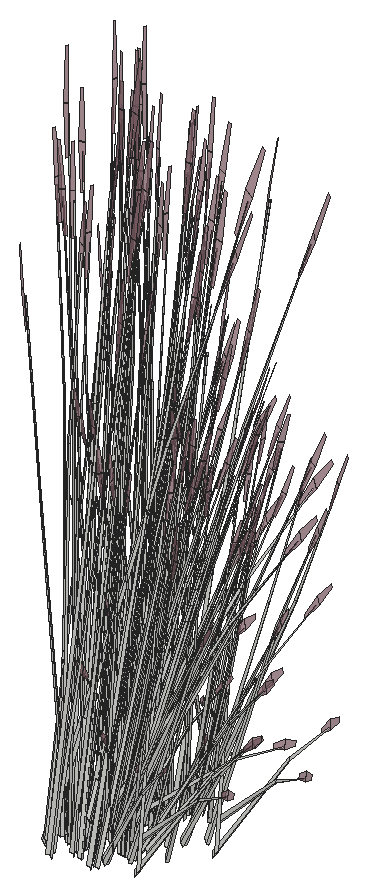
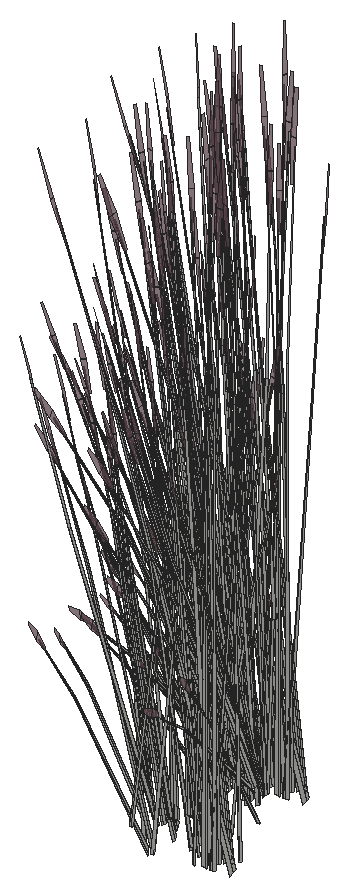
# SketchUp Ruby script. Lengths in inches.
U = 1.inch
M = Sketchup.active_model
def pt(a) = Geom::Point3d.new(a.map { |v| v * U })
def face(e, loops, mat)
  f = e.add_face(loops[0].map { |a| pt(a) })
  loops[1..].each { |l| e.add_face(l.map { |a| pt(a) }).erase! }
  f.material = f.back_material = mat if mat
  f
end
# faces: each face lists its corners as indices into pts; further lists are holes
def faces(e, pts, list, mat = nil) = list.each { |f| face(e, (f[0].is_a?(Array) ? f : [f]).map { |l| l.map { |i| pts[i] } }, mat) }
# xy, xz, yz: faces in a plane at the given z, y or x. An outline is a flat list of corners, or four numbers for a rectangle; further outlines are holes
def ring(l) = l.size == 4 ? [[l[0], l[1]], [l[2], l[1]], [l[2], l[3]], [l[0], l[3]]] : l.each_slice(2).to_a
def flat(e, list, mat, &to3) = list.each { |f| face(e, (f[0].is_a?(Array) ? f : [f]).map { |l| ring(l).map { |u, v| to3.(u, v) } }, mat) }
def xy(e, z, list, mat = nil) = flat(e, list, mat) { |x, y| [x, y, z] }
def xz(e, y, list, mat = nil) = flat(e, list, mat) { |x, z| [x, y, z] }
def yz(e, x, list, mat = nil) = flat(e, list, mat) { |y, z| [x, y, z] }
def lines(e, pts, list) = list.each { |a, b| e.add_line(pt(pts[a]), pt(pts[b])) }
# prism: a flat outline (further loops are holes) pulled along v
def prism(e, loops, v, mat = nil)
  f = face(e, loops, mat); d = Geom::Vector3d.new(v.map { |x| x * U })
  f.pushpull(f.normal.samedirection?(d) ? d.length : -d.length)
end
def box(e, o, s, mat = nil) = prism(e, [[o, [o[0] + s[0], o[1], o[2]], [o[0] + s[0], o[1] + s[1], o[2]], [o[0], o[1] + s[1], o[2]]]], [0, 0, s[2]], mat)
def at(x, y, z, deg = 0) = Geom::Transformation.translation(pt([x, y, z])) * Geom::Transformation.rotation(ORIGIN, Z_AXIS, deg.degrees)
def axes(o, x, y, z) = Geom::Transformation.new([*x, 0, *y, 0, *z, 0, *pt(o).to_a, 1])
def part(name) = M.definitions.add(name)
# library, detail: a bought-in or finely detailed component or shape, given as its bounding box
def library(name, o, s) = part(name).tap { |d| box(d.entities, o, s) }
def detail(e, o, s) = box(e.add_group.entities, o, s)
def put(e, d, t, mat = nil) = e.add_instance(d, t).tap { |i| i.material = mat if mat }
def group(e, t, mat = nil) = e.add_group.tap { |g| g.transformation = t; g.material = mat if mat }.entities
root = M.entities
M.materials.add("LightPink_Translucent").color = [144, 107, 117]
M.materials["LightPink_Translucent"].alpha = 0.75
c1 = part("blade")
p = [[2.15,0.21,22],[0,0.17,0],[0.09,0.45,0],[2.18,0.31,22],[2.29,0.31,22],[0.38,0.45,0],
  [2.48,0.24,33],[2.49,0.24,33],[2.48,0.22,33]]
faces(c1.entities,p,[[0,1,2,3],[4,5,2,3],[6,3,4,7],[8,0,3,6]])
c2 = part("seeds")
p = [[0.3,-0.1,1.38],[-0.01,-0.03,1.59],[-0.01,-0.03,0.03],[0.14,-0.07,-0.07],[0.29,-0.03,3],[0.15,0.01,3.11]]
faces(c2.entities,p,[[0,1,2,3],[1,0,4,5]],"LightPink_Translucent")
c3 = part("blade with seeds")
put(c3.entities,c1,at(0,0,0))
put(c3.entities,c2,axes([2.4,0.25,30.99],[1.5799,-0.05474,1.17369],[-0.12525,1.92788,0.29478],[-0.07173,-0.02425,1.56792]))
put(root,c3,axes([343.58,165.07,4.3125],[0.83726,-0.32623,-0.49651],[0.50045,0.58498,0],[0.19069,-0.0743,1.57504]))
put(root,c3,axes([348.55,166.2,4.88],[-0.31959,-0.01933,1.43002],[-0.32741,-0.51843,-0.30754],[0.39262,-0.14666,0.61141]))
put(root,c3,axes([350.3,166.7,7],[-0.11685,-0.00496,1.77383],[-0.48522,-0.53096,-0.16761],[0.19486,-0.17458,0.31391]))
put(root,c3,axes([344.57,166.41,4.35],[0.60257,-0.49041,-0.62353],[0.74854,0.44469,-0.16365],[0.24146,-0.12234,1.37633]))
put(root,c3,axes([348.92,165.25,5.06],[-0.29798,0.33213,1.1486],[-0.25612,-0.44624,0.84392],[0.24611,-0.11182,0.25299]))
put(root,c3,axes([348.49,166.5,6.82],[0.77872,-0.09325,-0.35414],[0.20563,0.53305,0.4572],[0.22316,-0.14318,0.87481]))
put(root,c3,axes([343.53,167.27,4.5],[0.43405,-0.58792,-0.44739],[0.90188,0.28295,0.21531],[0,-0.13553,1.43643]))
put(root,c3,axes([343.92,166.98,4.96],[-0.10425,-0.7445,-0.29095],[1.08575,-0.04502,-0.50002],[0.19119,-0.09917,1.59708]))
put(root,c3,axes([347.86,166.8125,7.34],[-0.77872,0.09325,0.35414],[-0.20563,-0.53305,-0.4572],[0.22316,-0.14318,0.87481]))
put(root,c3,axes([343.78,165.33,4.32],[0.83462,0.16144,-0.30978],[-0.21015,0.56852,0.30978],[0.16826,-0.06556,1.38974]))
put(root,c3,axes([348.5625,166.73,7.02],[0.61415,0.2744,0.0643],[-0.35756,0.39076,0.50621],[0.1969,-0.12633,0.77189]))
put(root,c3,axes([348.39,166.61,7.03],[0.22187,0.60049,0.48003],[-0.87033,0.10422,0.3958],[0.25651,-0.14123,0.9933]))
put(root,c3,axes([350.74,167.34,7.01],[0.12414,-0.09938,1.74944],[-0.15889,-0.60963,-0.27667],[0.31148,-0.11559,0.14031]))
put(root,c3,axes([344.0625,167.5625,4.73],[1.00799,0.31623,0.24065],[-0.48511,0.65709,0.50002],[0,-0.15147,1.60543]))
put(root,c3,axes([343.74,167.125,5.01],[-0.97146,0.04028,0.44739],[-0.08785,-0.66859,-0.21531],[0.17391,-0.06776,1.43643]))
put(root,c3,axes([348.29,168.26,7.33],[-0.45012,-0.59081,-0.1216],[0.79888,-0.29033,-0.67495],[0.33665,-0.07795,1.02557]))
put(root,c3,axes([348.26,167.76,6.97],[0.24236,-0.59349,-0.51099],[0.83094,0.20343,-0.3958],[0.33455,-0.05442,0.97773]))
put(root,c3,axes([346.94,165.34,4.67],[0.55932,-0.6538,0],[0.93577,0.36461,-0.51607],[0.21313,0.08304,1.63711]))
put(root,c3,axes([343.7,167.36,4.65],[0.38895,0.72959,0.45755],[-1.11135,0.2537,0.17955],[0.01358,-0.13406,1.58856]))
put(root,c3,axes([349.14,167.92,4.28],[-0.57619,0.0783,1.41583],[-0.09171,-0.62326,0.08104],[0.40356,-0.09434,0.80566]))
put(root,c3,axes([350.19,167.37,4.55],[-0.55463,-0.41721,-0.06488],[0.60744,-0.38228,-0.29416],[0.17212,-0.02691,0.97024]))
put(root,c3,axes([345.1,167.43,4.5],[0,-0.75495,0],[1.11865,0,0],[0,0,1.79456]))
put(root,c3,axes([346.46,165.68,4.77],[-0.83726,-0.32623,0.49651],[0.50045,-0.58498,0],[0.19069,0.0743,1.57504]))
put(root,c3,axes([348.1,167.97,7.27],[0.78611,-0.28816,-0.71045],[0.4381,0.59317,0.08574],[0.37982,-0.06738,1.00501]))
put(root,c3,axes([344.57,166.95,4.65],[-0.74176,0.59212,0.45755],[-0.88124,-0.52269,0.17955],[0.17882,-0.05909,1.58856]))
put(root,c3,axes([343.29,165.98,4.77],[-0.25843,0.64844,0.17642],[-0.9457,-0.1835,0.35086],[0.16336,-0.00316,1.60407]))
put(root,c3,axes([347.98,168.09,7.34],[-0.74348,-0.18202,0.35414],[0.21685,-0.53102,-0.4572],[0.29933,-0.04869,0.87481]))
put(root,c3,axes([342.89,166.5,3.89],[-0.88056,0.26122,1.28929],[-0.28027,-0.74951,0.50096],[0.54072,0.01247,1.46642]))
put(root,c3,axes([345.26,166.7,4.91],[0.17258,-0.58229,0.1448],[0.84319,0.10108,-0.41347],[0.15345,0.05979,1.26744]))
put(root,c3,axes([349.77,167.52,3.79],[-0.04675,-0.09906,1.76342],[0.32428,-0.57943,-0.26939],[0.32711,-0.00833,0.30037]))
put(root,c3,axes([344.9,166.85,5.01],[-0.53742,-0.54764,0.44739],[0.81403,-0.38564,-0.21531],[0.17391,0.06776,1.43643]))
put(root,c3,axes([345.17,166.89,4.96],[0.90324,-0.43318,-0.29095],[0.60064,0.61207,-0.50002],[0.22285,0.06216,1.59708]))
put(root,c3,axes([348.76,168.03,6.82],[0.74348,0.18202,-0.35414],[-0.21685,0.53102,0.4572],[0.29933,-0.04869,0.87481]))
put(root,c3,axes([347.45,165.73,4.3125],[0.83726,0.32623,-0.49651],[-0.50045,0.58498,0],[0.19069,0.0743,1.57504]))
put(root,c3,axes([345.86,167.59,4.5],[1.00089,0,0],[0,0.67548,0],[0,0,1.78407]))
put(root,c3,axes([346.15,166.01,4.77],[-0.96132,0.17317,0.17642],[-0.23737,-0.64447,0.35086],[0.08574,0.0939,1.60407]))
put(root,c3,axes([346.74,167.37,6.17],[-0.37107,0.01478,1.71376],[0.24616,-0.64047,0.13857],[0.5288,0.03961,0.73262]))
put(root,c3,axes([347.22,165.98,4.32],[0.21015,0.56852,-0.30978],[-0.83462,0.16144,0.30978],[0.16826,0.06556,1.38974]))
put(root,c3,axes([348.66,168.25,7.02],[0.32857,0.44488,0.0643],[-0.59916,0.21775,0.50621],[0.26412,-0.04296,0.77189]))
put(root,c3,axes([346.1,173.3,2.59],[-0.25429,0.13207,1.43002],[-0.76157,-0.23115,-0.30754],[0.14117,-0.28747,0.61141]))
put(root,c3,axes([345.54,167.25,4.67],[-1.13071,-0.13747,0.49198],[0.23011,-0.77639,0.19306],[0.16524,0.07497,1.70813]))
put(root,c3,axes([348.59,168.09,7.03],[-0.25275,0.59491,0.48003],[-0.83094,-0.20343,0.3958],[0.32677,-0.03575,0.9933]))
put(root,c3,axes([344.64,169.17,4.5],[-0.29189,-0.56252,0],[0.83351,-0.19699,0],[0,0,1.54371]))
put(root,c3,axes([345.73,169.09,4.48],[0.93921,-0.22138,-0.19198],[0.33003,0.6377,0.00008],[0.10367,-0.02447,1.73897]))
put(root,c3,axes([345.84,167.88,4.51],[0.62448,0.42144,0],[-0.62448,0.42144,0],[0,0,1.69266]))
put(root,c3,axes([347.53,167.7,4.77],[-0.70288,-0.47526,0.17642],[0.70832,-0.46097,0.35086],[-0.07763,0.09706,1.60407]))
put(root,c3,axes([346.23,166.98,4.35],[0.9306,0.10697,-0.62353],[-0.19638,0.65984,-0.16365],[0.27771,0.07995,1.37633]))
put(root,c3,axes([350.34,168.14,5.06],[-0.55274,0.10771,1.1486],[0.26018,-0.44517,0.84392],[0.29323,0.03046,0.25299]))
put(root,c3,axes([346.72,174.28,4.98],[0.02328,-0.60353,-0.71045],[0.98022,0.04053,0.08574],[0.10344,-0.25568,1.00501]))
put(root,c3,axes([348.09,173.34,4.72],[-0.00864,-0.12985,1.74944],[-0.72937,-0.3753,-0.27667],[0.11277,-0.2275,0.14031]))
put(root,c3,axes([345.62,173.97,3.875],[-0.16657,0.22426,1.71376],[-0.69879,-0.4641,0.13857],[0.31524,-0.28926,0.73262]))
put(root,c3,axes([347.89,172.87,4.71],[-0.09085,0.04984,1.77383],[-0.89014,-0.16814,-0.16761],[-0.03222,-0.21748,0.31391]))
put(root,c3,axes([345.83,167.39,5.01],[0.43405,-0.58792,0.44739],[0.90188,0.28295,-0.21531],[0,0.13553,1.43643]))
put(root,c3,axes([350.09,170.02,7],[-0.08089,-0.05712,1.77383],[0.17695,-0.61228,-0.16761],[0.31864,-0.03912,0.31391]))
put(root,c3,axes([345.16,172.25,2.77],[0.11476,0.38047,1.1486],[-0.63664,-0.21072,0.84392],[0.06851,-0.19481,0.25299]))
put(root,c3,axes([345.67,167.73,4.59],[0,0.75458,-0.05637],[-1.11865,0,0],[0,0.02371,1.79368]))
put(root,c3,axes([345.75,167.19,4.5],[0.53742,0.54764,-0.44739],[-0.81403,0.38564,0.21531],[0.17391,0.06776,1.43643]))
put(root,c3,axes([349.38,169.51,6.22],[-0.17122,-0.54847,-0.03492],[0.80929,-0.12609,-0.15832],[0.169,0.03477,0.52218]))
put(root,c3,axes([346.52,174.08,4.68],[-0.64041,-0.4384,-0.51099],[0.67652,-0.38394,-0.3958],[0.09744,-0.22274,0.97773]))
put(root,c3,axes([347.28,169.49,7.33],[0.0479,-0.66354,-0.1216],[0.90696,0.01814,-0.67495],[0.3493,0.04609,1.02557]))
put(root,c3,axes([348.11,167.72,4.77],[0,-0.65246,0.49651],[1.00089,0,0],[0,0.1486,1.57504]))
put(root,c3,axes([346.21,167.53,4.91],[0.83351,-0.19028,0.1448],[0.29189,0.54335,-0.41347],[0,0.11958,1.26744]))
put(root,c3,axes([347.14,169.23,7.34],[-0.50902,-0.40851,0.35414],[0.58122,-0.38671,-0.4572],[0.29531,0.05884,0.87481]))
put(root,c3,axes([345.12,173.43,4.73],[0.88151,0.17057,0.48003],[-0.30143,0.56078,0.3958],[-0.05297,-0.22053,0.9933]))
put(root,c3,axes([349.31,168.85,4.88],[-0.21545,-0.16047,1.43002],[0.28033,-0.53085,-0.30754],[0.43591,0.07191,0.61141]))
put(root,c3,axes([347.19,174.31,5.03],[-0.98321,-0.03233,-0.1216],[0.02687,-0.61208,-0.67495],[0.0683,-0.23574,1.02557]))
put(root,c3,axes([347.12,173.92,4.53],[0.60531,-0.34352,-0.35414],[0.573,0.39225,0.4572],[0.08718,-0.19929,0.87481]))
put(root,c3,axes([345.35,173.38,4.73],[0.6592,-0.22175,0.0643],[0.32265,0.40436,0.50621],[-0.06366,-0.17825,0.77189]))
put(root,c3,axes([345.45,169.43,4.5],[0.90188,0.29293,0],[-0.43405,0.60866,0],[0,0,1.74954]))
put(root,c3,axes([348.07,169.09,7.01],[0.19191,-0.01103,1.74944],[0.52639,-0.5069,-0.27667],[0.34136,0.06691,0.14031]))
put(root,c3,axes([347.33,169.17,7.27],[0.89428,0.01571,-0.71045],[-0.06006,0.66153,0.08574],[0.37886,0.06981,1.00501]))
put(root,c3,axes([347.88,173.71,1.49],[-0.1339,-0.0514,1.76342],[-0.34394,-0.57425,-0.26939],[0.23202,-0.15583,0.30037]))
put(root,c3,axes([345.13,169.1875,4.58],[0.38895,0.74956,-0.06012],[-1.11135,0.26265,0],[0.01358,0.02618,1.72173]))
put(root,c3,axes([348.79,167.83,4.67],[1.11865,0,0],[0,0.72922,-0.51607],[0,0.16609,1.63711]))
put(root,c3,axes([347.12,174.05,4.73],[0.63704,0.44518,0.48003],[-0.67652,0.38394,0.3958],[0.11751,-0.20886,0.9933]))
put(root,c3,axes([347.36,174.09,4.73],[0.73517,0.0304,0.0643],[-0.02016,0.45906,0.50621],[0.07693,-0.17585,0.77189]))
put(root,c3,axes([348.34,168.2,4.49],[-1.1181,-0.00522,-0.04976],[0,-0.72922,0.49943],[-0.03514,0.166,1.58352]))
put(root,c3,axes([345.92,167.57,4.96],[1.00749,0.31132,-0.29095],[-0.48511,0.65709,-0.50002],[0.03166,0.16133,1.59708]))
put(root,c3,axes([347.87,169.45,6.82],[0.50902,0.40851,-0.35414],[-0.58122,0.38671,0.4572],[0.29531,0.05884,0.87481]))
put(root,c3,axes([348.11,168.31,4.32],[-0.62448,0.40708,-0.30978],[-0.62448,-0.40708,0.30978],[0,0.13112,1.38974]))
put(root,c3,axes([346.81,174.4,5.05],[-0.60531,0.34352,0.35414],[-0.573,-0.39225,-0.4572],[0.08718,-0.19929,0.87481]))
put(root,c3,axes([347.61,169.6,7.02],[-0.04505,0.49615,0.0643],[-0.68022,-0.0136,0.50621],[0.26056,0.05192,0.77189]))
put(root,c3,axes([347.875,175.33,4.98],[0.4673,-0.51481,-0.71045],[0.81887,0.36587,0.08574],[0.27902,-0.18652,1.00501]))
put(root,c3,axes([345.81,168.06,4.5],[-0.43405,0.58792,-0.44739],[-0.90188,-0.28295,0.21531],[0,0.13553,1.43643]))
put(root,c3,axes([342.82,173.83,2.375],[-0.55932,-0.6538,0],[0.93577,-0.36461,-0.51607],[0.21313,-0.08304,1.63711]))
put(root,c3,axes([347.85,175.09,4.68],[-0.22982,-0.59576,-0.51099],[0.87033,-0.10422,-0.3958],[0.24941,-0.16002,0.97773]))
put(root,c3,axes([347.67,169.44,7.03],[-0.65964,0.42992,0.48003],[-0.5689,-0.45657,0.3958],[0.30948,0.0793,0.9933]))
put(root,c3,axes([348.26,175.51,5.03],[-0.82753,-0.35977,-0.1216],[0.47675,-0.52101,-0.67495],[0.2338,-0.18111,1.02557]))
put(root,c3,axes([345.57,169.94,7.34],[-0.13817,-0.52554,0.35414],[0.78985,-0.13877,-0.4572],[0.21215,0.1506,0.87481]))
put(root,c3,axes([348.54,168.32,4.3125],[0,0.65246,-0.49651],[-1.00089,0,0],[0,0.1486,1.57504]))
put(root,c3,axes([346.04,168.4,6.17],[-0.3323,-0.11241,1.71376],[0.68769,-0.4716,0.13857],[0.42861,0.21275,0.73262]))
put(root,c3,axes([343.58,173.73,2.02],[0.83726,-0.32623,-0.49651],[0.50045,0.58498,0],[0.19069,-0.0743,1.57504]))
put(root,c3,axes([348.55,174.85,2.59],[-0.31959,-0.01933,1.43002],[-0.32741,-0.51843,-0.30754],[0.39262,-0.14666,0.61141]))
put(root,c3,axes([350.3,175.36,4.71],[-0.11685,-0.00496,1.77383],[-0.48522,-0.53096,-0.16761],[0.19486,-0.17458,0.31391]))
put(root,c3,axes([346.1,166.92,6.77],[-0.77304,-0.33901,1.38283],[0.81626,-0.52782,0.59665],[0.24941,0.31809,1.33663]))
put(root,c3,axes([344.57,175.07,2.06],[0.60257,-0.49041,-0.62353],[0.74854,0.44469,-0.16365],[0.24146,-0.12234,1.37633]))
put(root,c3,axes([348.92,173.9,2.77],[-0.29798,0.33213,1.1486],[-0.25612,-0.44624,0.84392],[0.24611,-0.11182,0.25299]))
put(root,c3,axes([347.27,169.68,5.06],[-0.5037,-0.18761,1.1486],[0.6504,-0.19062,0.84392],[0.17543,0.16147,0.25299]))
put(root,c3,axes([345.5,170.21,7.33],[0.53309,-0.55848,-0.1216],[0.77201,0.32175,-0.67495],[0.26836,0.15779,1.02557]))
put(root,c3,axes([348.49,175.15,4.53],[0.77872,-0.09325,-0.35414],[0.20563,0.53305,0.4572],[0.22316,-0.14318,0.87481]))
put(root,c3,axes([343.53,175.93,2.21],[0.43405,-0.58792,-0.44739],[0.90188,0.28295,0.21531],[0,-0.13553,1.43643]))
put(root,c3,axes([344.8,170.68,7],[0.00265,-0.07899,1.77383],[0.76665,-0.34851,-0.16761],[0.2663,0.12439,0.31391]))
put(root,c3,axes([343.92,175.63,2.67],[-0.10425,-0.7445,-0.29095],[1.08575,-0.04502,-0.50002],[0.19119,-0.09917,1.59708]))
put(root,c3,axes([347.41,170.375,3.79],[0.06518,-0.0942,1.76342],[0.82057,-0.27742,-0.26939],[0.24877,0.14358,0.30037]))
put(root,c3,axes([346.33,168.24,4.39],[0.32803,0.59738,-0.69212],[-0.94492,0.21515,-0.18165],[0.03626,0.20229,1.52773]))
put(root,c3,axes([346.13,169.9375,6.97],[0.88277,-0.1551,-0.51099],[0.15442,0.58737,-0.3958],[0.23711,0.16832,0.97773]))
put(root,c3,axes([347.86,175.46,5.05],[-0.77872,0.09325,0.35414],[-0.20563,-0.53305,-0.4572],[0.22316,-0.14318,0.87481]))
put(root,c3,axes([343.68,170.02,7.34],[0.2697,-0.50175,0.35414],[0.78684,0.14635,-0.4572],[0.07215,0.20201,0.87481]))
put(root,c3,axes([343.78,173.99,2.03],[0.83462,0.16144,-0.30978],[-0.21015,0.56852,0.30978],[0.16826,-0.06556,1.38974]))
put(root,c3,axes([347.35,170.53,4.96],[-0.57368,-0.02046,1.0506],[0.37886,-0.43461,0.58006],[0.22663,0.15441,0.8241]))
put(root,c3,axes([345.7,170.42,7.02],[-0.4066,0.41448,0.0643],[-0.57901,-0.24131,0.50621],[0.18719,0.13288,0.77189]))
put(root,c3,axes([344.74,171.81,7.9375],[0.61821,-0.37431,-0.06488],[0.56645,0.40995,-0.29416],[0.03988,0.11616,0.97024]))
put(root,c3,axes([345.87,170.3,7.03],[-0.88979,0.14973,0.48003],[-0.15442,-0.58737,0.3958],[0.20926,0.17311,0.9933]))
put(root,c3,axes([348.5625,175.38,4.73],[0.61415,0.2744,0.0643],[-0.35756,0.39076,0.50621],[0.1969,-0.12633,0.77189]))
put(root,c3,axes([348.39,175.26,4.73],[0.22187,0.60049,0.48003],[-0.87033,0.10422,0.3958],[0.25651,-0.14123,0.9933]))
put(root,c3,axes([350.74,175.99,4.72],[0.12414,-0.09938,1.74944],[-0.15889,-0.60963,-0.27667],[0.31148,-0.11559,0.14031]))
put(root,c3,axes([345.48,169.48,4.88],[0.01579,-0.21629,1.43002],[0.75442,-0.24159,-0.30754],[0.23289,0.25887,0.61141]))
put(root,c3,axes([343.42,170.24,7.33],[0.87543,-0.30377,-0.1216],[0.4302,0.53915,-0.67495],[0.1155,0.2272,1.02557]))
put(root,c3,axes([344.0625,176.22,2.43],[1.00799,0.31623,0.24065],[-0.48511,0.65709,0.50002],[0,-0.15147,1.60543]))
put(root,c3,axes([343.58,170.35,3.79],[0.14478,-0.0355,1.76342],[0.8709,0.19542,-0.26939],[0.02547,0.22025,0.30037]))
put(root,c3,axes([343.74,175.78,2.72],[-0.97146,0.04028,0.44739],[-0.08785,-0.66859,-0.21531],[0.17391,-0.06776,1.43643]))
put(root,c3,axes([348.29,176.92,5.03],[-0.45012,-0.59081,-0.1216],[0.79888,-0.29033,-0.67495],[0.33665,-0.07795,1.02557]))
put(root,c3,axes([348.26,176.41,4.68],[0.24236,-0.59349,-0.51099],[0.83094,0.20343,-0.3958],[0.33455,-0.05442,0.97773]))
put(root,c3,axes([346.94,173.99,2.375],[0.55932,-0.6538,0],[0.93577,0.36461,-0.51607],[0.21313,0.08304,1.63711]))
put(root,c3,axes([344.17,170.21,6.97],[0.87941,0.16356,-0.51099],[-0.30143,0.56078,-0.3958],[0.08064,0.22578,0.97773]))
put(root,c3,axes([344.67,169.05,6.17],[-0.2045,-0.20949,1.71376],[0.94495,-0.17636,0.13857],[0.21357,0.32887,0.73262]))
put(root,c3,axes([343.7,176.02,2.36],[0.38895,0.72959,0.45755],[-1.11135,0.2537,0.17955],[0.01358,-0.13406,1.58856]))
put(root,c3,axes([349.14,176.58,1.98],[-0.57619,0.0783,1.41583],[-0.09171,-0.62326,0.08104],[0.40356,-0.09434,0.80566]))
put(root,c3,axes([350.19,176.03,2.26],[-0.55463,-0.41721,-0.06488],[0.60744,-0.38228,-0.29416],[0.17212,-0.02691,0.97024]))
put(root,c3,axes([343.77,170.55,6.82],[-0.2697,0.50175,-0.35414],[-0.78684,-0.14635,0.4572],[0.07215,0.20201,0.87481]))
put(root,c3,axes([345.1,176.08,2.21],[0,-0.75495,0],[1.11865,0,0],[0,0,1.79456]))
put(root,c3,axes([346.46,174.34,2.48],[-0.83726,-0.32623,0.49651],[0.50045,-0.58498,0],[0.19069,0.0743,1.57504]))
put(root,c3,axes([348.1,176.625,4.98],[0.78611,-0.28816,-0.71045],[0.4381,0.59317,0.08574],[0.37982,-0.06738,1.00501]))
put(root,c3,axes([344.57,175.6,2.36],[-0.74176,0.59212,0.45755],[-0.88124,-0.52269,0.17955],[0.17882,-0.05909,1.58856]))
put(root,c3,axes([346.1,180.47,4.88],[-0.25429,0.13207,1.43002],[-0.76157,-0.23115,-0.30754],[0.14117,-0.28747,0.61141]))
put(root,c3,axes([343.29,174.63,2.47],[-0.25843,0.64844,0.17642],[-0.9457,-0.1835,0.35086],[0.16336,-0.00316,1.60407]))
put(root,c3,axes([347.98,176.74,5.05],[-0.74348,-0.18202,0.35414],[0.21685,-0.53102,-0.4572],[0.29933,-0.04869,0.87481]))
put(root,c3,axes([343.85,170.1,7.27],[0.42698,0.53052,-0.71045],[-0.87893,0.29566,0.08574],[0.09984,0.25633,1.00501]))
put(root,c3,axes([342.89,175.15,1.59],[-0.88056,0.26122,1.28929],[-0.28027,-0.74951,0.50096],[0.54072,0.01247,1.46642]))
put(root,c3,axes([345.26,175.35,2.62],[0.17258,-0.58229,0.1448],[0.84319,0.10108,-0.41347],[0.15345,0.05979,1.26744]))
put(root,c3,axes([349.77,176.17,1.49],[-0.04675,-0.09906,1.76342],[0.32428,-0.57943,-0.26939],[0.32711,-0.00833,0.30037]))
put(root,c3,axes([343.21,171.44,7.01],[0.1134,0.10507,1.74944],[0.91515,0.04128,-0.27667],[0.09203,0.23172,0.14031]))
put(root,c3,axes([344.9,175.5,2.72],[-0.53742,-0.54764,0.44739],[0.81403,-0.38564,-0.21531],[0.17391,0.06776,1.43643]))
put(root,c3,axes([346.72,181.45,7.27],[0.02328,-0.60353,-0.71045],[0.98022,0.04053,0.08574],[0.10344,-0.25568,1.00501]))
put(root,c3,axes([348.09,180.5,7.01],[-0.00864,-0.12985,1.74944],[-0.72937,-0.3753,-0.27667],[0.11277,-0.2275,0.14031]))
